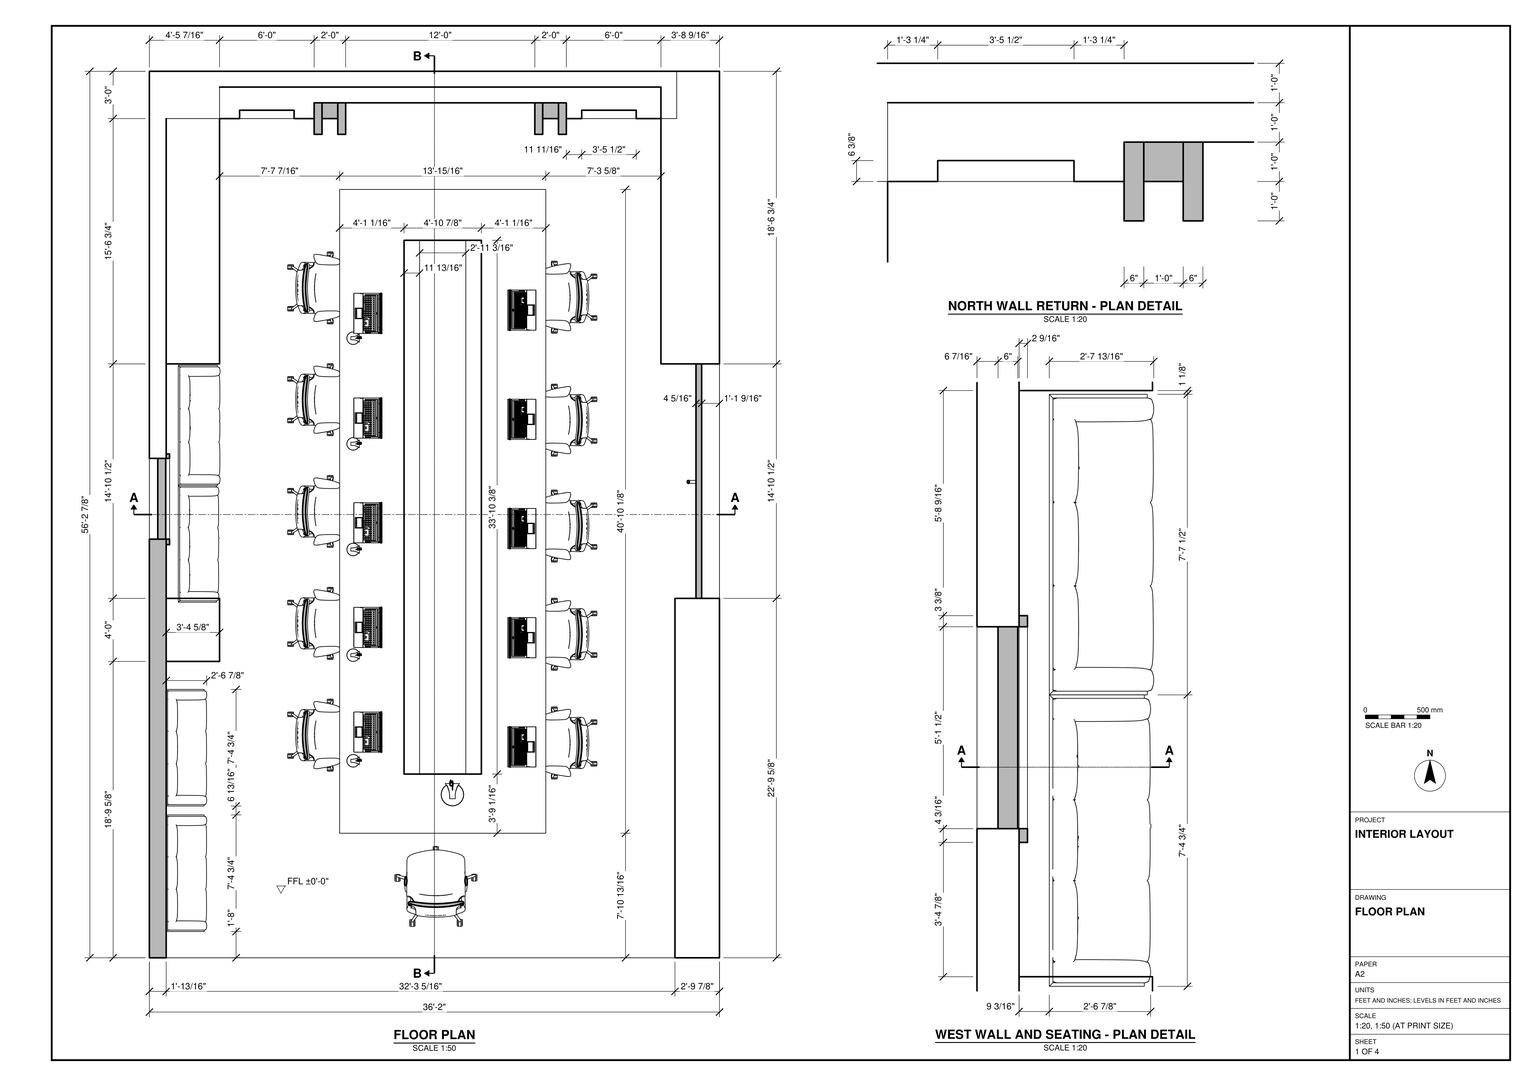
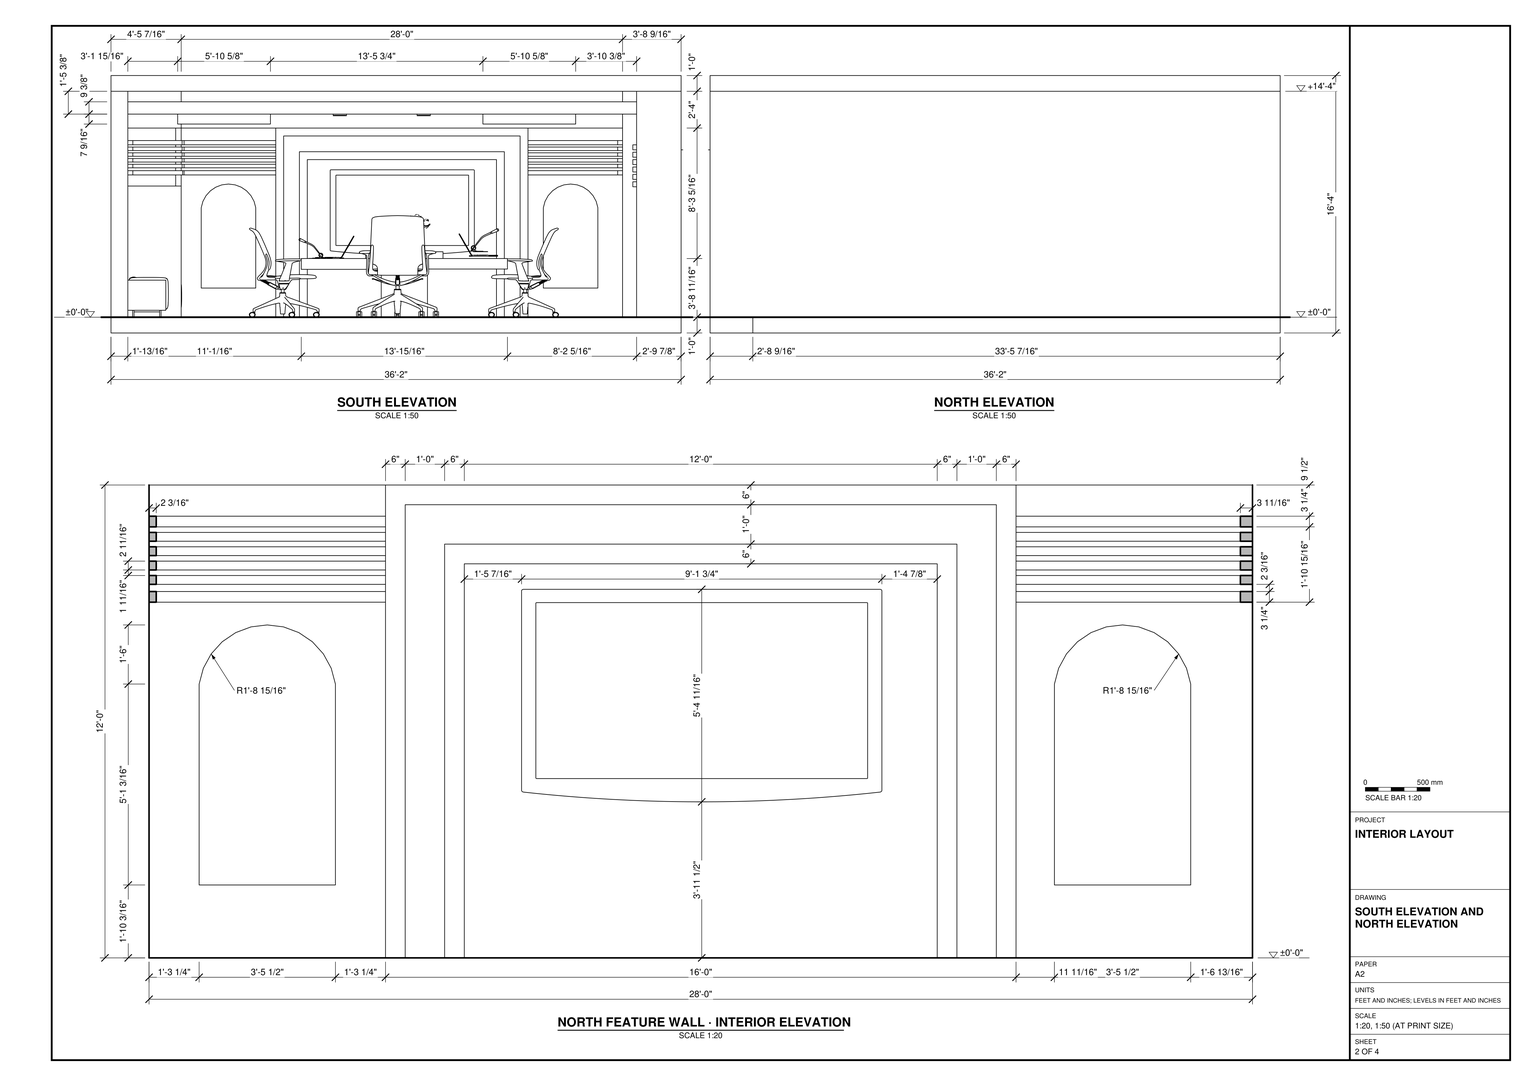
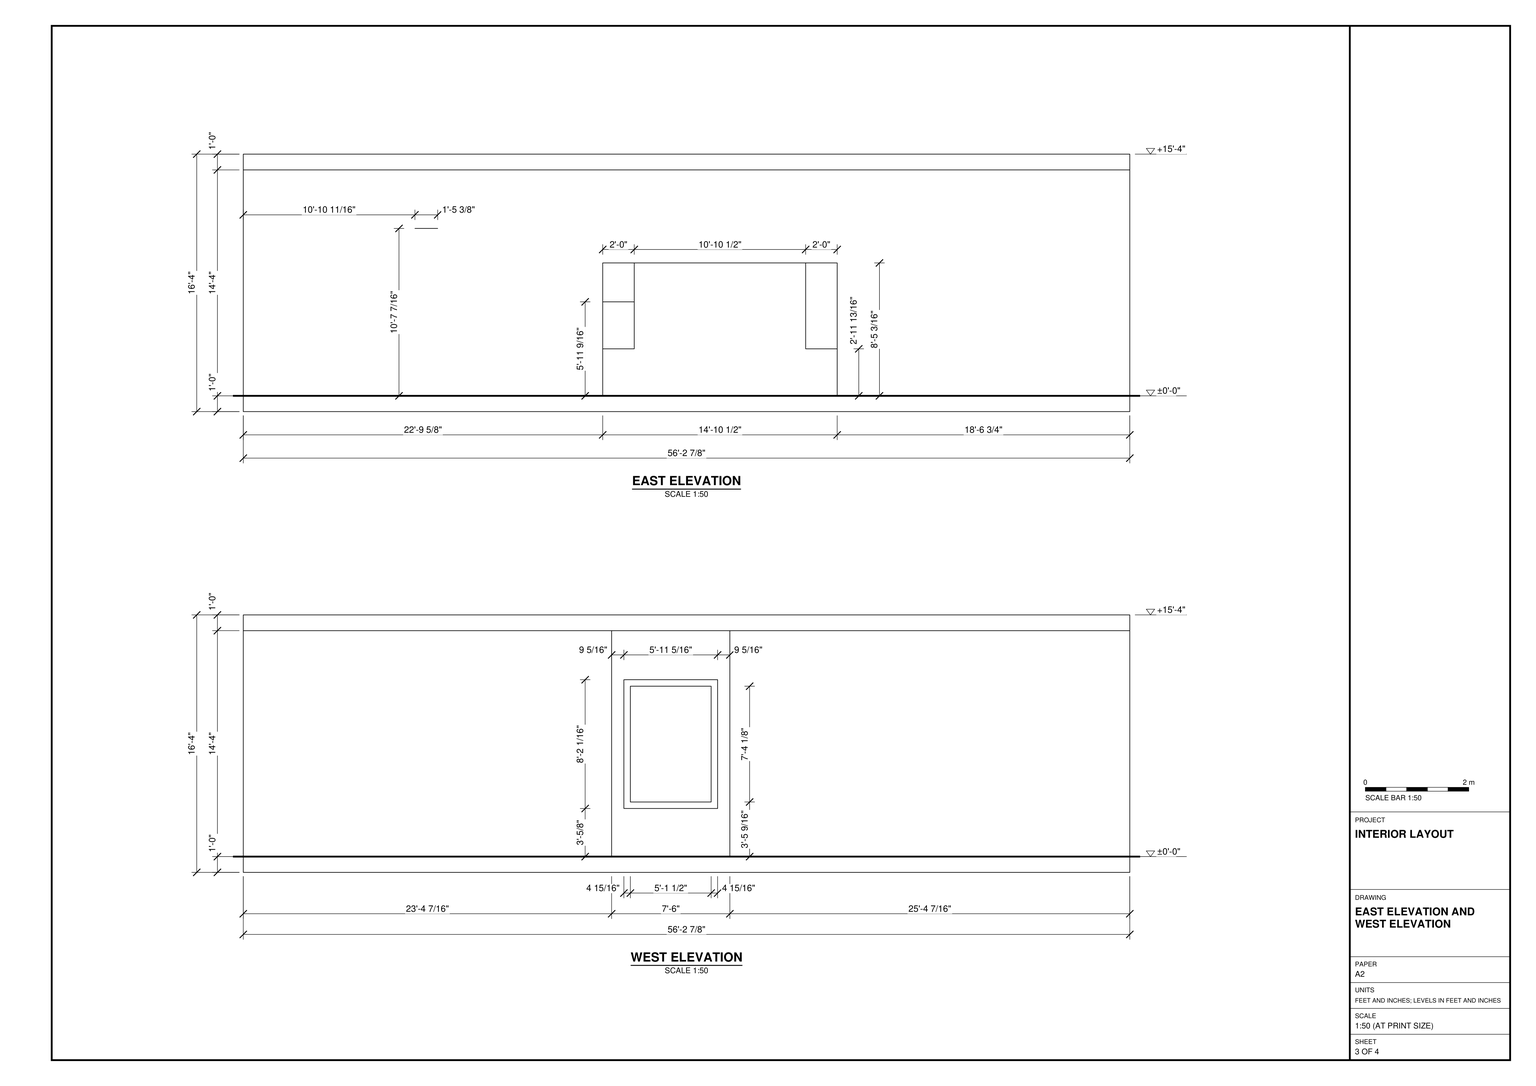
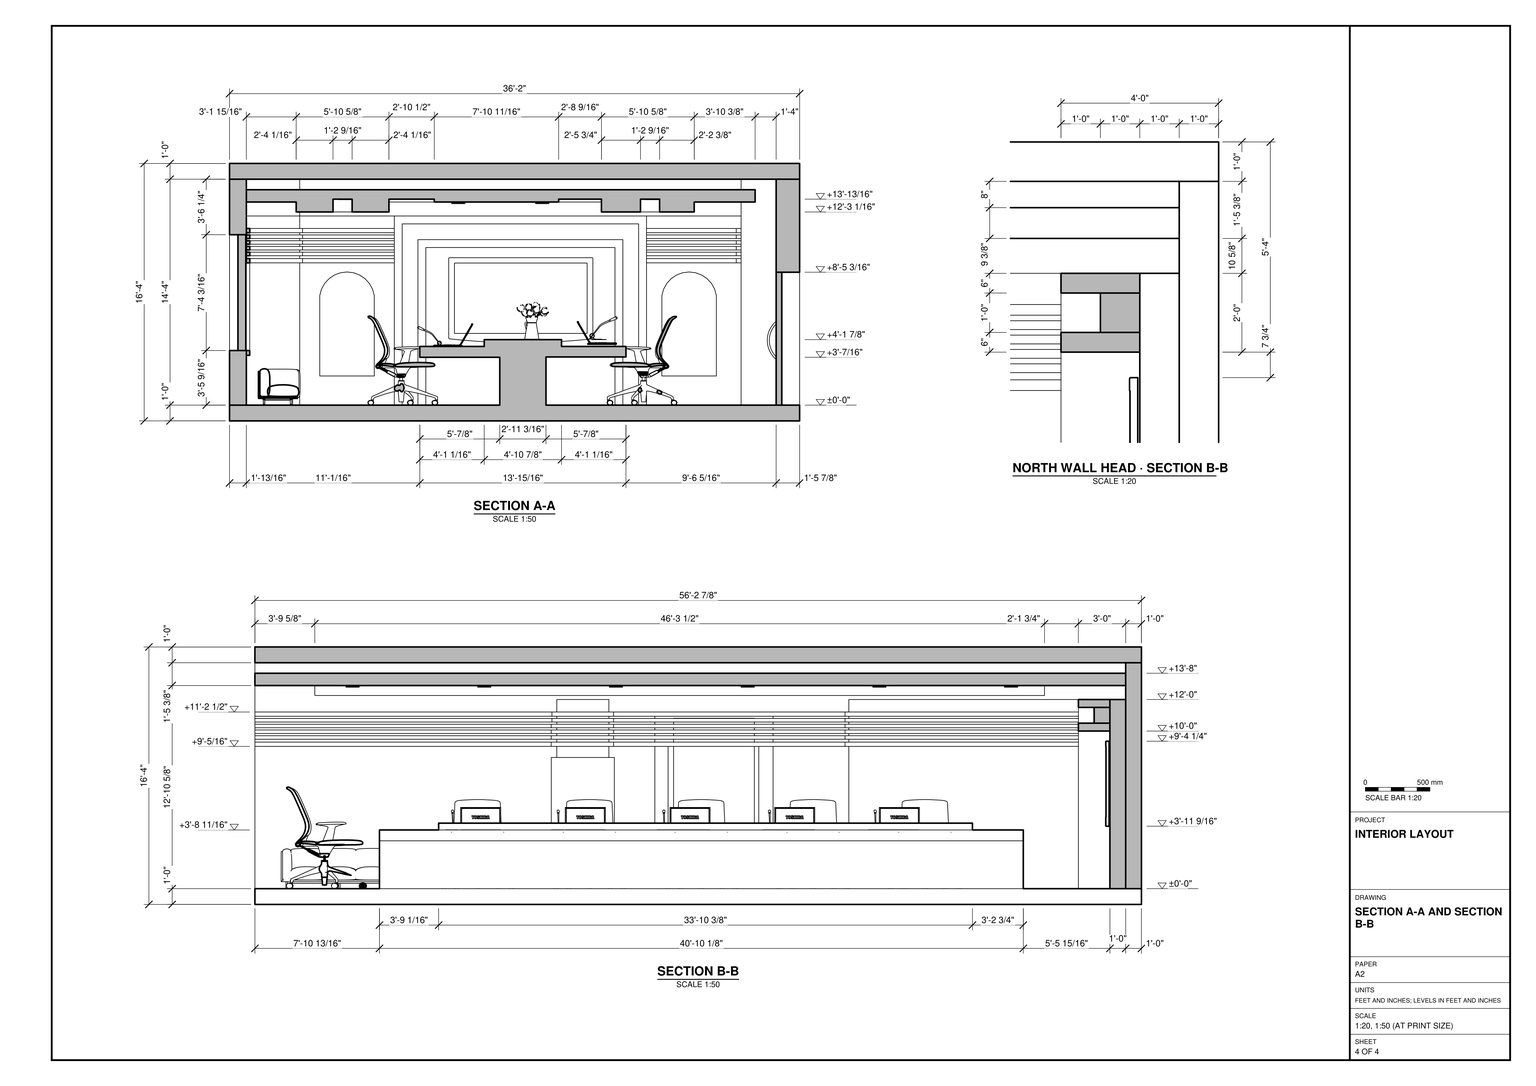
Build the meeting room in SketchUp using task_files/diagram_01.pdf. Work in feet and inches. Set the finished floor at ±0'-0" and make the overall model 36'-2" east to west, 56'-2 7/8" north to south and 16'-4" high, including the floor and overhead slabs.

Use the plan to set out the wall thicknesses and returns. Match the wide east wall opening and the raised, framed opening in the west wall to their respective elevations. On the inside of the north wall, build the stepped rectangular surround for the display. Include the arch-headed panels to either side and the horizontal slats above them.

Place the long meeting table on the north–south axis with its narrower central strip set back from both ends. Arrange five chairs along each long side facing the workstations, with a further chair at the south end facing the display. Fit the sofas along the west wall, preserving the break between the two seating runs shown in plan. Decor and loose items, including computer equipment, may be any suitable library components, for example from 3D Warehouse.

Keep the walls, slabs and each furniture or joinery piece in separate groups or components, and use components for repeated parts. Save one SketchUp model as output_files/meeting_room_with_a_north_display_wall.skp.

# SketchUp Ruby script. Lengths in inches.
U = 1.inch
M = Sketchup.active_model
def pt(a) = Geom::Point3d.new(a.map { |v| v * U })
def face(e, loops, mat)
  f = e.add_face(loops[0].map { |a| pt(a) })
  loops[1..].each { |l| e.add_face(l.map { |a| pt(a) }).erase! }
  f.material = f.back_material = mat if mat
  f
end
# faces: each face lists its corners as indices into pts; further lists are holes
def faces(e, pts, list, mat = nil) = list.each { |f| face(e, (f[0].is_a?(Array) ? f : [f]).map { |l| l.map { |i| pts[i] } }, mat) }
# xy, xz, yz: faces in a plane at the given z, y or x. An outline is a flat list of corners, or four numbers for a rectangle; further outlines are holes
def ring(l) = l.size == 4 ? [[l[0], l[1]], [l[2], l[1]], [l[2], l[3]], [l[0], l[3]]] : l.each_slice(2).to_a
def flat(e, list, mat, &to3) = list.each { |f| face(e, (f[0].is_a?(Array) ? f : [f]).map { |l| ring(l).map { |u, v| to3.(u, v) } }, mat) }
def xy(e, z, list, mat = nil) = flat(e, list, mat) { |x, y| [x, y, z] }
def xz(e, y, list, mat = nil) = flat(e, list, mat) { |x, z| [x, y, z] }
def yz(e, x, list, mat = nil) = flat(e, list, mat) { |y, z| [x, y, z] }
def lines(e, pts, list) = list.each { |a, b| e.add_line(pt(pts[a]), pt(pts[b])) }
# prism: a flat outline (further loops are holes) pulled along v
def prism(e, loops, v, mat = nil)
  f = face(e, loops, mat); d = Geom::Vector3d.new(v.map { |x| x * U })
  f.pushpull(f.normal.samedirection?(d) ? d.length : -d.length)
end
def box(e, o, s, mat = nil) = prism(e, [[o, [o[0] + s[0], o[1], o[2]], [o[0] + s[0], o[1] + s[1], o[2]], [o[0], o[1] + s[1], o[2]]]], [0, 0, s[2]], mat)
def at(x, y, z, deg = 0) = Geom::Transformation.translation(pt([x, y, z])) * Geom::Transformation.rotation(ORIGIN, Z_AXIS, deg.degrees)
def axes(o, x, y, z) = Geom::Transformation.new([*x, 0, *y, 0, *z, 0, *pt(o).to_a, 1])
def part(name) = M.definitions.add(name)
# library, detail: a bought-in or finely detailed component or shape, given as its bounding box
def library(name, o, s) = part(name).tap { |d| box(d.entities, o, s) }
def detail(e, o, s) = box(e.add_group.entities, o, s)
def put(e, d, t, mat = nil) = e.add_instance(d, t).tap { |i| i.material = mat if mat }
def group(e, t, mat = nil) = e.add_group.tap { |g| g.transformation = t; g.material = mat if mat }.entities
root = M.entities
M.materials.add("[Roofing Slate Tan]").color = [198, 174, 127]
M.materials.add("[Translucent Glass Safety]").color = [204, 235, 244]
M.materials["[Translucent Glass Safety]"].alpha = 0.5
M.materials.add("[Wood Bamboo]").color = [170, 101, 41]
M.materials.add("[Wood Cherry Original]").color = [152, 86, 42]
M.materials.add("[Wood Floor Parquet]").color = [127, 77, 33]
c1 = library("of3",[-14.23,-14.05,0],[28.46,27.7,42.45])
c2 = library("Laptop ",[0,0,0],[208.6875,200.66,116.73])
c3 = part("Laptop")
put(c3.entities,c2,at(-0.1875,-132.375,0))
c4 = library("microfono+pc",[-14.125,-4.42,-0.59],[17.32,34.67,27.76])
c5 = library("Pitcher with flowers",[-0.57,-0.27,-0.17],[11.49,12.54,12.88])
c6 = library("Untitled",[82.71,28.87,-11.8125],[39.77,1.97,25.2])
c7 = library("Tlon Light 450 Ceiling 152 006",[-8.86,-8.86,-3.78],[17.72,17.72,3.56])
c8 = library("Group\#1",[0,0,0],[11.09,178.5,101.1875])
c9 = library("Group\#31",[0,0,0],[112.99,39.26,34.22])
xy(root,-12,[[0,0,401.4375,674.875],[401.4375,0,434,674.875]])
xy(root,0,[[0,0,12.8125,0,12.8125,638.875,53.4375,638.875,53.4375,662.875,389.4375,662.875,389.4375,638.875,401.4375,638.875,401.4375,674.875,0,674.875],[[12.8125,0,400.125,0,400.125,273.625,434,273.625,434,452.125,389.4375,452.125,389.4375,638.875,317.4375,638.875,317.4375,626.875,311.4375,626.875,311.4375,638.875,299.4375,638.875,299.4375,626.875,293.4375,626.875,293.4375,650.875,149.4375,650.875,149.4375,626.875,143.4375,626.875,143.4375,638.875,131.4375,638.875,131.4375,626.875,125.4375,626.875,125.4375,638.875,53.4375,638.875,53.4375,452.125,12.8125,452.125,12.8125,273.625,53.4375,273.625,53.4375,225.625,12.8125,225.625],[205.72,94.82,240.91,584.94]],[400.125,0,434,273.625],[12.8125,225.625,53.4375,273.625],[12.8125,452.125,53.4375,638.875],
  [389.4375,452.125,434,452.125,434,674.875,401.4375,674.875,401.4375,638.875,389.4375,638.875],[125.4375,626.875,131.4375,650.875],[143.4375,626.875,149.4375,650.875],[293.4375,626.875,299.4375,650.875],[311.4375,626.875,317.4375,650.875],
  [53.4375,638.875,125.4375,638.875,125.4375,650.875,317.4375,650.875,317.4375,638.875,389.4375,638.875,389.4375,662.875,53.4375,662.875],[131.4375,638.875,143.4375,650.875],[299.4375,638.875,311.4375,650.875]])
xy(root,22.2,[[68.6875,638.875,110.1875,645.25],[329.125,638.875,370.625,645.25]])
xy(root,36.4375,[[144.85,94.82,205.72,584.94]])
xy(root,36.6875,[[240.91,94.82,301.78,584.94]])
xy(root,37.95,[[12.8125,314.53,15.375,383.57]])
xy(root,41.57,[[0,318.71,12.8125,380.2],[12.8125,318.71,15.375,380.2]])
xy(root,44.6875,[[[144.85,94.82,301.78,584.94],[193.89,139.86,252.75,546.22]]],"[Wood Floor Parquet]")
xy(root,49.875,[[193.89,139.86,252.75,546.22]])
xy(root,99.3125,[[397.25,0.6875,400.125,273.625]])
xy(root,99.875,[[12.8125,225.625,53.4375,225.625,53.4375,273.625,12.8125,273.625,12.8125,269.4375,49.25,269.4375,49.25,229.8125,12.8125,229.8125]],"[Wood Floor Parquet]")
xy(root,101.1875,[[416.125,273.625,434,452.125]])
xy(root,103.125,[[397.25,0.6875,400.125,273.625]])
xy(root,104.9375,[[397.25,0,400.125,273.625]])
xy(root,108.3125,[[12.8125,0,12.8125,229.8125,49.25,229.8125,49.25,269.4375,12.8125,269.4375,12.8125,314.53,15.375,314.53,15.375,318.71,12.8125,318.71,12.8125,380.2,15.375,380.2,15.375,383.57,12.8125,383.57,12.8125,452.125,53.4375,452.125,53.4375,638.875,55.625,638.875,55.625,449.25,15.4375,449.25,15.4375,273.0625,54.5625,273.0625,54.5625,225.5625,16.64,225.5625,16.64,0],[12.8125,314.53,15.375,318.71],[385.75,452.125,385.75,634.875,317.4375,634.875,317.4375,638.875,389.4375,638.875,389.4375,452.125],[55.625,634.875,125.4375,638.875]])
xy(root,108.75,[[397.25,0,400.125,273.625]])
xy(root,110.5625,[[397.25,0,400.125,273.625]])
xy(root,111.5625,[[12.8125,0,16.64,0,16.64,225.5625,54.5625,225.5625,54.5625,273.0625,15.4375,273.0625,15.4375,449.25,55.625,449.25,55.625,638.875,53.4375,638.875,53.4375,452.125,12.8125,452.125,12.8125,269.4375,49.25,269.4375,49.25,229.8125,12.8125,229.8125],[385.75,452.125,389.4375,452.125,389.4375,638.875,317.4375,638.875,317.4375,634.875,385.75,634.875],[55.625,634.875,125.4375,638.875]])
xy(root,113.75,[[12.8125,0,12.8125,229.8125,49.25,229.8125,49.25,269.4375,12.8125,269.4375,12.8125,452.125,53.4375,452.125,53.4375,638.875,55.625,638.875,55.625,449.25,15.4375,449.25,15.4375,273.0625,54.125,273.0625,54.125,225.5625,16.64,225.5625,16.64,0],[385.75,452.125,385.75,634.875,317.4375,634.875,317.4375,638.875,389.4375,638.875,389.4375,452.125],[55.625,634.875,125.4375,638.875]])
xy(root,114.375,[[397.25,0,400.125,273.625]])
xy(root,116.1875,[[397.25,0,400.125,273.625]])
xy(root,116.4375,[[12.8125,0,16.64,0,16.64,225.5625,54.125,225.5625,54.125,273.0625,15.4375,273.0625,15.4375,449.25,55.625,449.25,55.625,638.875,53.4375,638.875,53.4375,452.125,12.8125,452.125,12.8125,269.4375,49.25,269.4375,49.25,229.8125,12.8125,229.8125],[385.75,452.125,389.4375,452.125,389.4375,638.875,317.4375,638.875,317.4375,634.875,385.75,634.875],[55.625,634.875,125.4375,638.875]])
xy(root,118.125,[[12.8125,0,12.8125,229.8125,49.25,229.8125,49.25,269.4375,12.8125,269.4375,12.8125,452.125,53.4375,452.125,53.4375,638.875,55.625,638.875,55.625,449.25,15.4375,449.25,15.4375,273.0625,54.125,273.0625,54.125,225.5625,16.64,225.5625,16.64,0],[385.75,452.125,385.75,634.875,317.4375,634.875,317.4375,638.875,389.4375,638.875,389.4375,452.125],[55.625,634.875,125.4375,638.875]])
xy(root,120,[[397.25,0,400.125,273.625]])
xy(root,120,[[149.4375,626.875,293.4375,650.875]],"[Wood Floor Parquet]")
xy(root,120.8125,[[12.8125,0,16.64,0,16.64,225.5625,54.125,225.5625,54.125,273.0625,15.4375,273.0625,15.4375,449.25,55.625,449.25,55.625,638.875,53.4375,638.875,53.4375,452.125,12.8125,452.125,12.8125,269.4375,49.25,269.4375,49.25,229.8125,12.8125,229.8125],[385.75,452.125,389.4375,452.125,389.4375,638.875,317.4375,638.875,317.4375,634.875,385.75,634.875],[55.625,634.875,125.4375,638.875]])
xy(root,121.8125,[[397.25,0,400.125,273.625]])
xy(root,122.5,[[12.8125,0,12.8125,229.8125,49.25,229.8125,49.25,269.4375,12.8125,269.4375,12.8125,452.125,53.4375,452.125,53.4375,638.875,55.625,638.875,55.625,449.25,15.4375,449.25,15.4375,273.0625,54.125,273.0625,54.125,225.5625,16.64,225.5625,16.64,0],[385.75,452.125,385.75,634.875,317.4375,634.875,317.4375,638.875,389.4375,638.875,389.4375,452.125],[55.625,634.875,125.4375,638.875]])
xy(root,125.1875,[[12.8125,0,16.64,0,16.64,225.5625,54.125,225.5625,54.125,273.0625,15.4375,273.0625,15.4375,449.25,55.625,449.25,55.625,638.875,53.4375,638.875,53.4375,452.125,12.8125,452.125,12.8125,269.4375,49.25,269.4375,49.25,229.8125,12.8125,229.8125],[385.75,452.125,389.4375,452.125,389.4375,638.875,317.4375,638.875,317.4375,634.875,385.75,634.875],[55.625,634.875,125.4375,638.875]])
xy(root,125.625,[[397.25,0,400.125,273.625]])
xy(root,126,[[143.4375,638.875,299.4375,650.875]])
xy(root,126,[[143.4375,626.875,299.4375,638.875]],"[Wood Floor Parquet]")
xy(root,126.875,[[12.8125,0,12.8125,229.8125,49.25,229.8125,49.25,269.4375,12.8125,269.4375,12.8125,452.125,53.4375,452.125,53.4375,638.875,55.625,638.875,55.625,449.25,15.4375,449.25,15.4375,273.0625,54.125,273.0625,54.125,226.125,16.64,226.125,16.64,0],[385.75,452.125,385.75,634.875,317.4375,634.875,317.4375,638.875,389.4375,638.875,389.4375,452.125],[55.625,634.875,125.4375,638.875]])
xy(root,127.4375,[[397.25,0,400.125,273.625]])
xy(root,129.5625,[[12.8125,0,16.64,0,16.64,226.125,54.125,226.125,54.125,273.0625,15.4375,273.0625,15.4375,449.25,55.625,449.25,55.625,638.875,53.4375,638.875,53.4375,452.125,12.8125,452.125,12.8125,269.4375,49.25,269.4375,49.25,229.8125,12.8125,229.8125],[385.75,452.125,389.4375,452.125,389.4375,638.875,317.4375,638.875,317.4375,634.875,385.75,634.875],[55.625,634.875,125.4375,638.875]])
xy(root,129.74,[[0,318.71,12.8125,380.2]])
xy(root,131.25,[[12.8125,0,12.8125,229.8125,49.25,229.8125,49.25,269.4375,12.8125,269.4375,12.8125,452.125,53.4375,452.125,53.4375,638.875,55.625,638.875,55.625,449.25,15.4375,449.25,15.4375,273.0625,54.125,273.0625,54.125,226.125,16.64,226.125,16.64,0],[397.25,0,400.125,273.625],[385.75,452.125,385.75,634.875,317.4375,634.875,317.4375,638.875,389.4375,638.875,389.4375,452.125],[55.625,634.875,125.4375,638.875]])
xy(root,134.5,[[12.8125,0,16.64,0,16.64,226.125,54.125,226.125,54.125,273.0625,15.4375,273.0625,15.4375,449.25,55.625,449.25,55.625,638.875,53.4375,638.875,53.4375,452.125,12.8125,452.125,12.8125,269.4375,49.25,269.4375,49.25,229.8125,12.8125,229.8125],[385.75,452.125,389.4375,452.125,389.4375,638.875,317.4375,638.875,317.4375,634.875,385.75,634.875],[55.625,634.875,125.4375,638.875]])
xy(root,138,[[131.4375,626.875,311.4375,638.875],[131.4375,638.875,311.4375,650.875]])
xy(root,144,[[125.4375,626.875,317.4375,650.875]])
xy(root,144,[[12.8125,229.8125,49.25,269.4375],[12.8125,452.125,53.4375,452.125,53.4375,638.875,125.4375,638.875,125.4375,650.875,317.4375,650.875,317.4375,638.875,389.4375,638.875,389.4375,662.875,12.8125,662.875]],"[Wood Floor Parquet]")
xy(root,147.0625,[[[50.75,45.59,121.375,601.09],[78.79,73.64,93.33,251.05],[78.79,312.76,93.33,490.18]],[[283.125,45.59,353.75,601.09],[312.86,312.76,327.39,490.18],[312.86,73.64,327.39,251.05]]])
xy(root,154.625,[[[12.8125,0,400.125,662.875],[50.75,45.59,155.875,601.09],[250.5625,45.59,353.75,601.09]]])
xy(root,156.8125,[[121.375,45.59,155.875,601.09],[250.5625,45.59,283.125,601.09],[78.79,73.64,93.33,251.05],[312.86,73.64,327.39,251.05],[78.79,312.76,93.33,490.18],
  [312.86,312.76,327.39,490.18]],"[Wood Floor Parquet]")
xy(root,164,[[12.8125,0,400.125,662.875]])
xy(root,172,[[0,0,0,674.875,434,674.875,434,0,400.125,0,400.125,273.625,416.125,273.625,416.125,452.125,389.4375,452.125,389.4375,662.875,12.8125,662.875,12.8125,0],[12.8125,0,12.8125,662.875,389.4375,662.875,389.4375,452.125,416.125,452.125,416.125,273.625,400.125,273.625,400.125,0]])
xy(root,184,[[0,0,434,674.875]])
xz(root,0,[[0,-12,434,0],[0,0,12.8125,172],[400.125,0,434,172],[397.25,104.9375,400.125,108.75],[12.8125,108.3125,16.64,111.5625],
  [397.25,110.5625,400.125,114.375],[12.8125,113.75,16.64,116.4375],[397.25,116.1875,400.125,120],[12.8125,118.125,16.64,120.8125],[397.25,121.8125,400.125,125.625],
  [12.8125,122.5,16.64,125.1875],[12.8125,126.875,16.64,129.5625],[397.25,127.4375,400.125,131.25],[12.8125,131.25,16.64,134.5],[12.8125,154.625,400.125,164],
  [0,172,434,184]])
xz(root,0.6875,[[397.25,99.3125,400.125,103.125]])
xz(root,45.59,[[50.75,147.0625,121.375,154.625],[283.125,147.0625,353.75,154.625],[121.375,154.625,155.875,156.8125],[250.5625,154.625,283.125,156.8125]])
xz(root,73.64,[[78.79,147.0625,93.33,156.8125],[312.86,147.0625,327.39,156.8125]])
xz(root,94.82,[[205.72,0,240.91,0,240.91,36.6875,301.78,36.6875,301.78,44.6875,144.85,44.6875,144.85,36.4375,205.72,36.4375]],"[Wood Floor Parquet]")
xz(root,139.86,[[193.89,44.6875,252.75,49.875]])
xz(root,225.5625,[[16.64,108.3125,54.5625,111.5625],[16.64,113.75,54.125,116.4375],[16.64,118.125,54.125,120.8125],[16.64,122.5,54.125,125.1875]])
xz(root,225.625,[[12.8125,0,53.4375,99.875]],"[Wood Floor Parquet]")
xz(root,226.125,[[16.64,126.875,54.125,129.5625],[16.64,131.25,54.125,134.5]])
xz(root,229.8125,[[12.8125,111.5625,49.25,113.75],[12.8125,116.4375,49.25,118.125],[12.8125,120.8125,49.25,122.5],[12.8125,125.1875,49.25,126.875],[12.8125,129.5625,49.25,131.25]])
xz(root,229.8125,[[12.8125,99.875,49.25,108.3125],[12.8125,134.5,49.25,144]],"[Wood Floor Parquet]")
xz(root,251.05,[[78.79,147.0625,93.33,156.8125],[312.86,147.0625,327.39,156.8125]],"[Wood Floor Parquet]")
xz(root,269.4375,[[12.8125,99.875,49.25,108.3125],[12.8125,111.5625,49.25,113.75],[12.8125,116.4375,49.25,118.125],[12.8125,120.8125,49.25,122.5],[12.8125,125.1875,49.25,126.875],
  [12.8125,129.5625,49.25,131.25],[12.8125,134.5,49.25,144]])
xz(root,273.0625,[[15.4375,108.3125,54.5625,111.5625],[15.4375,113.75,54.125,116.4375],[15.4375,118.125,54.125,120.8125],[15.4375,122.5,54.125,125.1875],[15.4375,126.875,54.125,129.5625],
  [15.4375,131.25,54.125,134.5]])
xz(root,273.625,[[12.8125,0,53.4375,99.875],[400.125,0,400.125,172,416.125,172,416.125,101.1875,434,101.1875,434,0],[397.25,99.3125,400.125,103.125],[397.25,104.9375,400.125,108.75],[397.25,110.5625,400.125,114.375],
  [397.25,116.1875,400.125,120],[397.25,121.8125,400.125,125.625],[397.25,127.4375,400.125,131.25]])
xz(root,312.76,[[78.79,147.0625,93.33,156.8125],[312.86,147.0625,327.39,156.8125]])
xz(root,314.53,[[12.8125,37.95,15.375,108.3125]])
xz(root,318.71,[[0,41.57,12.8125,129.74],[12.8125,41.57,15.375,108.3125]])
xz(root,380.2,[[0,41.57,12.8125,129.74],[12.8125,41.57,15.375,108.3125]])
xz(root,383.57,[[12.8125,37.95,15.375,108.3125]])
xz(root,449.25,[[15.4375,108.3125,55.625,111.5625],[15.4375,113.75,55.625,116.4375],[15.4375,118.125,55.625,120.8125],[15.4375,122.5,55.625,125.1875],[15.4375,126.875,55.625,129.5625],
  [15.4375,131.25,55.625,134.5]])
xz(root,452.125,[[12.8125,108.3125,53.4375,111.5625],[385.75,108.3125,389.4375,111.5625],[12.8125,111.5625,53.4375,113.75],[12.8125,113.75,53.4375,116.4375],[385.75,113.75,389.4375,116.4375],
  [12.8125,116.4375,53.4375,118.125],[12.8125,118.125,53.4375,120.8125],[385.75,118.125,389.4375,120.8125],[12.8125,120.8125,53.4375,122.5],[12.8125,122.5,53.4375,125.1875],
  [385.75,122.5,389.4375,125.1875],[12.8125,125.1875,53.4375,126.875],[12.8125,126.875,53.4375,129.5625],[385.75,126.875,389.4375,129.5625],[12.8125,129.5625,53.4375,131.25],
  [12.8125,131.25,53.4375,134.5],[385.75,131.25,389.4375,134.5]])
xz(root,452.125,[[12.8125,0,53.4375,108.3125],[389.4375,0,434,0,434,101.1875,416.125,101.1875,416.125,172,389.4375,172],[12.8125,134.5,53.4375,144]],"[Wood Floor Parquet]")
xz(root,490.18,[[78.79,147.0625,93.33,156.8125],[312.86,147.0625,327.39,156.8125]],"[Wood Floor Parquet]")
xz(root,546.22,[[193.89,44.6875,252.75,49.875]])
xz(root,584.94,[[205.72,0,205.72,36.4375,144.85,36.4375,144.85,44.6875,301.78,44.6875,301.78,36.6875,240.91,36.6875,240.91,0]])
xz(root,601.09,[[50.75,147.0625,121.375,154.625],[283.125,147.0625,353.75,154.625]])
xz(root,601.09,[[121.375,154.625,155.875,156.8125],[250.5625,154.625,283.125,156.8125]],"[Wood Floor Parquet]")
xz(root,626.875,[[125.4375,0,131.4375,0,131.4375,138,311.4375,138,311.4375,0,317.4375,0,317.4375,144,125.4375,144]])
xz(root,626.875,[[143.4375,0,149.4375,0,149.4375,120,293.4375,120,293.4375,0,299.4375,0,299.4375,126,143.4375,126]],"[Wood Floor Parquet]")
xz(root,634.875,[[55.625,108.3125,125.4375,111.5625],[317.4375,108.3125,385.75,111.5625],[55.625,113.75,125.4375,116.4375],[317.4375,113.75,385.75,116.4375],[55.625,118.125,125.4375,120.8125],
  [317.4375,118.125,385.75,120.8125],[55.625,122.5,125.4375,125.1875],[317.4375,122.5,385.75,125.1875],[55.625,126.875,125.4375,129.5625],[317.4375,126.875,385.75,129.5625],
  [55.625,131.25,125.4375,134.5],[317.4375,131.25,385.75,134.5]])
xz(root,638.875,[[53.4375,108.3125,55.625,111.5625],[53.4375,111.5625,125.4375,113.75],[317.4375,111.5625,389.4375,113.75],[53.4375,113.75,55.625,116.4375],[53.4375,116.4375,125.4375,118.125],
  [317.4375,116.4375,389.4375,118.125],[53.4375,118.125,55.625,120.8125],[53.4375,120.8125,125.4375,122.5],[317.4375,120.8125,389.4375,120.8125,389.4375,122.5,317.125,122.5,317.125,125.1875,389.4375,125.1875,389.4375,126.875,317.4375,126.875],[53.4375,122.5,55.625,125.1875],
  [317.125,122.5,317.4375,125.1875],[53.4375,125.1875,125.4375,126.875],[53.4375,126.875,55.625,129.5625],[53.4375,129.5625,125.4375,131.25],[317.4375,129.5625,389.4375,131.25],
  [53.4375,131.25,55.625,134.5]])
xz(root,638.875,[[131.4375,0,143.4375,0,143.4375,126,299.4375,126,299.4375,0,311.4375,0,311.4375,138,131.4375,138]],"[Roofing Slate Tan]")
xz(root,638.875,[[[53.4375,0,125.4375,108.3125],[68.6875,22.2,68.6875,83.39,69.97,88.2,72.35,92.57,75.7,96.26,79.82,99.06,84.49,100.8,89.4375,101.39,94.38,100.8,99.05,99.06,103.17,96.26,106.52,92.57,108.9,88.2,110.1875,83.39,110.1875,22.2]],[[317.4375,0,389.4375,108.3125],[329.125,22.2,329.125,83.39,330.41,88.2,332.79,92.57,336.14,96.26,340.26,99.06,344.93,100.8,349.875,101.39,354.82,100.8,359.49,99.06,363.61,96.26,366.96,92.57,369.34,88.2,370.625,83.39,370.625,22.2]],[53.4375,134.5,125.4375,144],[317.4375,134.5,389.4375,144]],"[Wood Floor Parquet]")
xz(root,645.25,[[68.6875,22.2,110.1875,22.2,110.1875,83.39,108.9,88.2,106.52,92.57,103.17,96.26,99.05,99.06,94.38,100.8,89.4375,101.39,84.49,100.8,79.82,99.06,75.7,96.26,72.35,92.57,69.97,88.2,68.6875,83.39],[329.125,22.2,370.625,22.2,370.625,83.39,369.34,88.2,366.96,92.57,363.61,96.26,359.49,99.06,354.82,100.8,349.875,101.39,344.93,100.8,340.26,99.06,336.14,96.26,332.79,92.57,330.41,88.2,329.125,83.39]])
xz(root,650.875,[[125.4375,0,125.4375,144,317.4375,144,317.4375,0,311.4375,0,311.4375,138,131.4375,138,131.4375,0],[131.4375,0,131.4375,138,311.4375,138,311.4375,0,299.4375,0,299.4375,126,143.4375,126,143.4375,0],[143.4375,0,143.4375,126,299.4375,126,299.4375,0,293.4375,0,293.4375,120,149.4375,120,149.4375,0]])
xz(root,650.875,[[149.4375,0,293.4375,120]],"[Wood Cherry Original]")
xz(root,662.875,[[53.4375,0,389.4375,144],[12.8125,144,53.4375,154.625],[12.8125,154.625,53.4375,164],[389.4375,154.625,400.125,164],[12.8125,164,53.4375,172]])
xz(root,662.875,[[53.4375,144,389.4375,154.625],[53.4375,154.625,389.4375,164],[53.4375,164,389.4375,172]],"[Wood Floor Parquet]")
xz(root,674.875,[[0,-12,401.4375,0],[401.4375,-12,434,0],[0,0,434,172],[0,172,434,184]])
yz(root,0,[[0,-12,674.875,0],[0,0,304.46,172],[[304.46,0,394.46,172],[313.78,36.63,385.13,134.68]],[394.46,0,674.875,172],[[313.78,36.63,385.13,134.68],[318.71,41.57,380.2,129.74]],
  [0,172,674.875,184]])
yz(root,12.8125,[[225.625,0,225.625,99.875,229.8125,99.875,229.8125,144,269.4375,144,269.4375,134.5,273.625,134.5,273.625,131.25,269.4375,131.25,269.4375,129.5625,273.625,129.5625,273.625,126.875,269.4375,126.875,269.4375,125.1875,273.625,125.1875,273.625,122.5,269.4375,122.5,269.4375,120.8125,273.625,120.8125,273.625,118.125,269.4375,118.125,269.4375,116.4375,273.625,116.4375,273.625,113.75,269.4375,113.75,269.4375,111.5625,273.625,111.5625,273.625,108.3125,269.4375,108.3125,269.4375,99.875,273.625,99.875,273.625,0],[273.625,0,304.46,0,304.46,111.5625,273.625,111.5625,273.625,108.3125,304.46,108.3125,269.4375,108.3125,269.4375,99.875,273.625,99.875],[304.46,0,394.46,0,394.46,108.3125,383.57,108.3125,383.57,37.95,314.53,37.95,314.53,108.3125,304.46,108.3125],[452.125,0,638.875,144],[314.53,37.95,314.53,108.3125,318.71,108.3125,318.71,41.57,380.2,41.57,380.2,108.3125,383.57,108.3125,383.57,37.95],
  [304.46,108.3125,318.71,111.5625],[318.71,108.3125,380.2,111.5625],[380.2,108.3125,394.46,111.5625],[0,111.5625,229.8125,113.75],[269.4375,111.5625,304.46,113.75],
  [304.46,111.5625,318.71,113.75],[318.71,111.5625,380.2,113.75],[380.2,111.5625,394.46,113.75],[394.46,111.5625,452.125,113.75],[273.625,113.75,304.46,116.4375],
  [[273.625,113.75,452.125,113.75,452.125,116.4375,394.46,116.4375,394.46,118.125,452.125,118.125,452.125,120.8125,394.46,120.8125,394.46,122.5,452.125,122.5,452.125,125.1875,394.46,125.1875,394.46,126.875,452.125,126.875,452.125,129.5625,394.46,129.5625,394.46,131.25,304.46,131.25,304.46,129.5625,273.625,129.5625,273.625,126.875,304.46,126.875,304.46,125.1875,273.625,125.1875,273.625,122.5,304.46,122.5,304.46,120.8125,273.625,120.8125,273.625,118.125,304.46,118.125,304.46,116.4375,273.625,116.4375],[318.71,126.875,394.46,129.5625],[304.46,122.5,380.2,125.1875],[318.71,118.125,394.46,120.8125]],[304.46,113.75,318.71,116.4375],[318.71,113.75,380.2,116.4375],[380.2,113.75,394.46,116.4375],[394.46,113.75,452.125,116.4375],
  [0,116.4375,229.8125,118.125],[269.4375,116.4375,304.46,118.125],[304.46,116.4375,318.71,118.125],[318.71,116.4375,380.2,118.125],[380.2,116.4375,394.46,118.125],
  [394.46,116.4375,452.125,118.125],[273.625,118.125,304.46,120.8125],[304.46,118.125,318.71,120.8125],[318.71,118.125,380.2,120.8125],[318.71,118.125,380.2,122.5],
  [380.2,118.125,394.46,120.8125],[394.46,118.125,452.125,120.8125],[0,120.8125,229.8125,122.5],[269.4375,120.8125,304.46,122.5],[304.46,120.8125,318.71,122.5],
  [318.71,120.8125,380.2,122.5],[380.2,120.8125,394.46,122.5],[394.46,120.8125,452.125,122.5],[273.625,122.5,304.46,125.1875],[304.46,122.5,318.71,125.1875],
  [318.71,122.5,380.2,125.1875],[380.2,122.5,394.46,125.1875],[394.46,122.5,452.125,125.1875],[0,125.1875,229.8125,126.875],[269.4375,125.1875,304.46,126.875],
  [304.46,125.1875,318.71,126.875],[318.71,125.1875,380.2,126.875],[380.2,125.1875,394.46,126.875],[394.46,125.1875,452.125,126.875],[273.625,126.875,304.46,129.5625],
  [304.46,126.875,318.71,129.5625],[318.71,126.875,380.2,129.5625],[380.2,126.875,394.46,129.5625],[394.46,126.875,452.125,129.5625],[0,129.5625,229.8125,131.25],
  [269.4375,129.5625,304.46,131.25],[304.46,129.5625,318.71,129.5625,318.71,129.74,380.2,129.74,380.2,129.5625,394.46,129.5625,394.46,131.25,304.46,131.25],[318.71,129.5625,380.2,129.74],[394.46,129.5625,452.125,131.25],[273.625,131.25,304.46,134.5],
  [304.46,131.25,394.46,134.5],[394.46,131.25,452.125,134.5],[0,154.625,662.875,164]])
yz(root,12.8125,[[0,0,225.625,0,225.625,99.875,229.8125,99.875,229.8125,108.3125,0,108.3125],[394.46,0,452.125,0,452.125,108.3125,394.46,108.3125,452.125,108.3125,452.125,111.5625,394.46,111.5625],[0,134.5,229.8125,134.5,229.8125,144,269.4375,144,269.4375,134.5,452.125,134.5,452.125,144,662.875,144,662.875,154.625,0,154.625],[0,164,662.875,172]],"[Wood Floor Parquet]")
yz(root,15.375,[[314.53,37.95,383.57,37.95,383.57,108.3125,380.2,108.3125,380.2,41.57,318.71,41.57,318.71,108.3125,314.53,108.3125]])
yz(root,15.4375,[[273.0625,108.3125,449.25,111.5625],[273.0625,113.75,449.25,116.4375],[273.0625,118.125,449.25,120.8125],[273.0625,122.5,449.25,125.1875],[273.0625,126.875,449.25,129.5625],
  [273.0625,131.25,449.25,134.5]])
yz(root,16.64,[[0,108.3125,225.5625,111.5625],[0,113.75,225.5625,116.4375],[0,118.125,225.5625,120.8125],[0,122.5,225.5625,125.1875],[0,126.875,226.125,129.5625],
  [0,131.25,226.125,134.5]])
yz(root,49.25,[[229.8125,111.5625,269.4375,113.75],[229.8125,116.4375,269.4375,118.125],[229.8125,120.8125,269.4375,122.5],[229.8125,125.1875,269.4375,126.875],[229.8125,129.5625,269.4375,131.25]])
yz(root,49.25,[[229.8125,99.875,269.4375,108.3125],[229.8125,134.5,269.4375,144]],"[Wood Floor Parquet]")
yz(root,50.75,[[45.59,147.0625,601.09,154.625]])
yz(root,53.4375,[[452.125,108.3125,638.875,111.5625],[452.125,111.5625,638.875,113.75],[452.125,113.75,638.875,116.4375],[452.125,116.4375,638.875,118.125],[452.125,118.125,638.875,120.8125],
  [452.125,120.8125,638.875,122.5],[452.125,122.5,638.875,125.1875],[452.125,125.1875,638.875,126.875],[452.125,126.875,638.875,129.5625],[452.125,129.5625,638.875,131.25],
  [452.125,131.25,638.875,134.5]])
yz(root,53.4375,[[225.625,0,273.625,99.875],[452.125,0,638.875,108.3125],[452.125,134.5,638.875,144]],"[Wood Floor Parquet]")
yz(root,54.125,[[225.5625,113.75,273.0625,116.4375],[225.5625,118.125,273.0625,120.8125],[225.5625,122.5,273.0625,125.1875],[226.125,126.875,273.0625,129.5625],[226.125,131.25,273.0625,134.5]])
yz(root,54.5625,[[225.5625,108.3125,273.0625,111.5625]])
yz(root,55.625,[[449.25,108.3125,634.875,111.5625],[634.875,108.3125,638.875,111.5625],[449.25,113.75,634.875,116.4375],[634.875,113.75,638.875,116.4375],[449.25,118.125,634.875,120.8125],
  [634.875,118.125,638.875,120.8125],[449.25,122.5,634.875,125.1875],[634.875,122.5,638.875,125.1875],[449.25,126.875,634.875,129.5625],[634.875,126.875,638.875,129.5625],
  [449.25,131.25,634.875,134.5],[634.875,131.25,638.875,134.5]])
yz(root,68.6875,[[638.875,22.2,645.25,83.39]])
yz(root,78.79,[[73.64,147.0625,251.05,156.8125],[312.76,147.0625,490.18,156.8125]],"[Wood Floor Parquet]")
yz(root,93.33,[[73.64,147.0625,251.05,156.8125],[312.76,147.0625,490.18,156.8125]],"[Wood Floor Parquet]")
yz(root,110.1875,[[638.875,22.2,645.25,83.39]])
yz(root,121.375,[[45.59,147.0625,601.09,156.8125]])
yz(root,125.4375,[[626.875,0,626.875,144,638.875,144,638.875,134.5,634.875,134.5,634.875,131.25,638.875,131.25,638.875,129.5625,634.875,129.5625,634.875,126.875,638.875,126.875,638.875,125.1875,634.875,125.1875,634.875,122.5,638.875,122.5,638.875,120.8125,634.875,120.8125,634.875,118.125,638.875,118.125,638.875,116.4375,634.875,116.4375,634.875,113.75,638.875,113.75,638.875,111.5625,634.875,111.5625,634.875,108.3125,638.875,108.3125,638.875,0],[638.875,0,638.875,108.3125,634.875,108.3125,634.875,111.5625,638.875,111.5625,638.875,113.75,634.875,113.75,634.875,116.4375,638.875,116.4375,638.875,118.125,634.875,118.125,634.875,120.8125,638.875,120.8125,638.875,122.5,634.875,122.5,634.875,125.1875,638.875,125.1875,638.875,126.875,634.875,126.875,634.875,129.5625,638.875,129.5625,638.875,131.25,634.875,131.25,634.875,134.5,638.875,134.5,638.875,144,650.875,144,650.875,0]])
yz(root,131.4375,[[626.875,0,638.875,138],[638.875,0,650.875,138]])
yz(root,143.4375,[[638.875,0,650.875,126]])
yz(root,143.4375,[[626.875,0,638.875,126]],"[Wood Floor Parquet]")
yz(root,144.85,[[94.82,36.4375,584.94,44.6875]],"[Wood Floor Parquet]")
yz(root,149.4375,[[626.875,0,650.875,120]],"[Wood Floor Parquet]")
yz(root,155.875,[[45.59,154.625,601.09,156.8125]],"[Wood Floor Parquet]")
yz(root,193.89,[[139.86,44.6875,546.22,49.875]])
yz(root,205.72,[[94.82,0,584.94,36.4375]],"[Wood Floor Parquet]")
yz(root,240.91,[[94.82,0,584.94,36.6875]],"[Wood Floor Parquet]")
yz(root,250.5625,[[45.59,154.625,601.09,156.8125]],"[Wood Floor Parquet]")
yz(root,252.75,[[139.86,44.6875,546.22,49.875]])
yz(root,283.125,[[45.59,147.0625,601.09,156.8125]])
yz(root,293.4375,[[626.875,0,650.875,120]],"[Wood Floor Parquet]")
yz(root,299.4375,[[638.875,0,650.875,126]])
yz(root,299.4375,[[626.875,0,638.875,126]],"[Wood Floor Parquet]")
yz(root,301.78,[[94.82,36.6875,584.94,44.6875]],"[Wood Floor Parquet]")
yz(root,311.4375,[[626.875,0,638.875,138],[638.875,0,650.875,138]])
yz(root,312.86,[[73.64,147.0625,251.05,156.8125],[312.76,147.0625,490.18,156.8125]],"[Wood Floor Parquet]")
yz(root,317.4375,[[626.875,0,638.875,0,638.875,108.3125,634.875,108.3125,634.875,111.5625,638.875,111.5625,638.875,113.75,634.875,113.75,634.875,116.4375,638.875,116.4375,638.875,118.125,634.875,118.125,634.875,120.8125,638.875,120.8125,638.875,122.5,634.875,122.5,634.875,125.1875,638.875,125.1875,638.875,126.875,634.875,126.875,634.875,129.5625,638.875,129.5625,638.875,131.25,634.875,131.25,634.875,134.5,638.875,134.5,638.875,144,626.875,144],[638.875,0,650.875,0,650.875,144,638.875,144,638.875,134.5,634.875,134.5,634.875,131.25,638.875,131.25,638.875,129.5625,634.875,129.5625,634.875,126.875,638.875,126.875,638.875,120.8125,634.875,120.8125,634.875,118.125,638.875,118.125,638.875,116.4375,634.875,116.4375,634.875,113.75,638.875,113.75,638.875,111.5625,634.875,111.5625,634.875,108.3125,638.875,108.3125],[634.875,122.5,638.875,125.1875]])
yz(root,327.39,[[73.64,147.0625,251.05,156.8125],[312.76,147.0625,490.18,156.8125]],"[Wood Floor Parquet]")
yz(root,329.125,[[638.875,22.2,645.25,83.39]])
yz(root,353.75,[[45.59,147.0625,601.09,154.625]])
yz(root,370.625,[[638.875,22.2,645.25,83.39]])
yz(root,385.75,[[452.125,108.3125,634.875,111.5625],[452.125,113.75,634.875,116.4375],[452.125,118.125,634.875,120.8125],[452.125,122.5,634.875,125.1875],[452.125,126.875,634.875,129.5625],
  [452.125,131.25,634.875,134.5]])
yz(root,389.4375,[[638.875,0,638.875,108.3125,452.125,108.3125,452.125,111.5625,638.875,111.5625,638.875,113.75,452.125,113.75,452.125,116.4375,638.875,116.4375,638.875,118.125,452.125,118.125,452.125,120.8125,638.875,120.8125,638.875,122.5,452.125,122.5,452.125,125.1875,638.875,125.1875,638.875,126.875,452.125,126.875,452.125,129.5625,638.875,129.5625,638.875,131.25,452.125,131.25,452.125,134.5,638.875,134.5,638.875,144,662.875,144,662.875,0],[452.125,111.5625,638.875,113.75],[452.125,116.4375,638.875,118.125],[452.125,120.8125,638.875,122.5],[452.125,125.1875,638.875,126.875],
  [452.125,129.5625,638.875,131.25]])
yz(root,389.4375,[[452.125,0,638.875,108.3125],[452.125,134.5,452.125,172,662.875,172,662.875,144,638.875,144,638.875,134.5]],"[Wood Floor Parquet]")
yz(root,397.25,[[0.6875,99.3125,273.625,103.125],[0,104.9375,273.625,108.75],[0,110.5625,273.625,114.375],[0,116.1875,273.625,120],[0,121.8125,273.625,125.625],
  [0,127.4375,273.625,131.25]])
yz(root,400.125,[[0,99.3125,0.6875,103.125],[0.6875,99.3125,273.625,103.125],[0,103.125,273.625,104.9375],[0,104.9375,273.625,108.75],[0,108.75,273.625,110.5625],
  [0,110.5625,273.625,114.375],[0,114.375,273.625,116.1875],[0,116.1875,273.625,120],[0,120,273.625,121.8125],[0,121.8125,273.625,125.625],
  [0,125.625,273.625,127.4375],[0,127.4375,273.625,131.25],[0,154.625,273.625,164],[273.625,154.625,452.125,164],[452.125,154.625,662.875,164]])
yz(root,400.125,[[0,0,273.625,99.3125],[0,131.25,273.625,154.625],[0,164,273.625,172]],"[Wood Floor Parquet]")
yz(root,416.125,[[273.625,101.1875,452.125,172]],"[Wood Bamboo]")
yz(root,434,[[0,-12,674.875,0],[0,0,273.625,0,273.625,101.1875,452.125,101.1875,452.125,0,674.875,0,674.875,172,0,172],[0,172,674.875,184]])
p = [[69.97,638.875,88.2],[68.6875,638.875,83.39],[68.6875,645.25,83.39],[69.97,645.25,88.2],[110.1875,638.875,83.39],[108.9,638.875,88.2],
  [108.9,645.25,88.2],[110.1875,645.25,83.39],[330.41,638.875,88.2],[329.125,638.875,83.39],[329.125,645.25,83.39],[330.41,645.25,88.2],
  [370.625,638.875,83.39],[369.34,638.875,88.2],[369.34,645.25,88.2],[370.625,645.25,83.39],[72.35,638.875,92.57],[72.35,645.25,92.57],
  [106.52,638.875,92.57],[106.52,645.25,92.57],[332.79,638.875,92.57],[332.79,645.25,92.57],[366.96,638.875,92.57],[366.96,645.25,92.57],
  [75.7,638.875,96.26],[75.7,645.25,96.26],[103.17,638.875,96.26],[103.17,645.25,96.26],[336.14,638.875,96.26],[336.14,645.25,96.26],
  [363.61,638.875,96.26],[363.61,645.25,96.26],[79.82,638.875,99.06],[79.82,645.25,99.06],[99.05,638.875,99.06],[99.05,645.25,99.06],
  [340.26,638.875,99.06],[340.26,645.25,99.06],[359.49,638.875,99.06],[359.49,645.25,99.06],[84.49,638.875,100.8],[84.49,645.25,100.8],
  [94.38,638.875,100.8],[94.38,645.25,100.8],[344.93,638.875,100.8],[344.93,645.25,100.8],[354.82,638.875,100.8],[354.82,645.25,100.8],
  [89.4375,638.875,101.39],[89.4375,645.25,101.39],[349.875,638.875,101.39],[349.875,645.25,101.39],[416.23,130.68,127.4375],[416.23,148.05,127.4375],
  [400.83,148.05,127.4375],[400.83,130.68,127.4375],[435.33,130.66,127.4375],[435.33,148.02,127.4375],[419.93,148.02,127.4375],[419.93,130.66,127.4375]]
faces(root,p,[[0,1,2,3],[4,5,6,7],[8,9,10,11],[12,13,14,15],[16,0,3,17],[5,18,19,6],[20,8,11,21],[13,22,23,14],
  [24,16,17,25],[18,26,27,19],[28,20,21,29],[22,30,31,23],[32,24,25,33],[26,34,35,27],[36,28,29,37],[30,38,39,31],
  [40,32,33,41],[34,42,43,35],[44,36,37,45],[38,46,47,39],[48,40,41,49],[42,48,49,43],[50,44,45,51],[46,50,51,47]])
lines(root,p,[[52,53],[53,54],[54,55],[55,52],[56,57],[58,59],[59,56],[57,58]])
put(root,c1,axes([131.54,169.5,0],[0,1.92761,0],[-1.92761,0,0],[0,0,1.59884]))
put(root,c1,axes([131.54,254.62,0],[0,1.92761,0],[-1.92761,0,0],[0,0,1.59884]))
put(root,c1,axes([131.54,339.75,0],[0,1.92761,0],[-1.92761,0,0],[0,0,1.59884]))
put(root,c1,axes([131.54,424.87,0],[0,1.92761,0],[-1.92761,0,0],[0,0,1.59884]))
put(root,c1,axes([131.54,510,0],[0,1.92761,0],[-1.92761,0,0],[0,0,1.59884]))
put(root,c1,axes([314.42,163.55,0],[0,-1.92761,0],[1.92761,0,0],[0,0,1.59884]))
put(root,c1,axes([314.42,246.3,0],[0,-1.92761,0],[1.92761,0,0],[0,0,1.59884]))
put(root,c1,axes([314.42,328.68,0],[0,-1.92761,0],[1.92761,0,0],[0,0,1.59884]))
put(root,c1,axes([314.42,409.3,0],[0,-1.92761,0],[1.92761,0,0],[0,0,1.59884]))
put(root,c1,axes([314.42,502.93,0],[0,-1.92761,0],[1.92761,0,0],[0,0,1.59884]),"[Wood Floor Parquet]")
put(root,c3,axes([274.88,145.24,46.4],[0,0.147,0],[-0.147,0,0],[0,0,0.147]))
put(root,c3,axes([274.88,228.36,46.4],[0,0.147,0],[-0.147,0,0],[0,0,0.147]))
put(root,c3,axes([274.88,311.49,46.4],[0,0.147,0],[-0.147,0,0],[0,0,0.147]))
put(root,c3,axes([274.88,394.61,46.4],[0,0.147,0],[-0.147,0,0],[0,0,0.147]))
put(root,c3,axes([274.88,477.74,46.4],[0,0.147,0],[-0.147,0,0],[0,0,0.147]))
put(root,c3,axes([175.03,187.13,44.6875],[0,-0.147,0],[0.147,0,0],[0,0,0.147]))
put(root,c3,axes([175.03,266.82,44.6875],[0,-0.147,0],[0.147,0,0],[0,0,0.147]))
put(root,c3,axes([175.03,346.51,44.6875],[0,-0.147,0],[0.147,0,0],[0,0,0.147]))
put(root,c3,axes([175.03,426.19,44.6875],[0,-0.147,0],[0.147,0,0],[0,0,0.147]))
put(root,c3,axes([175.03,505.88,44.6875],[0,-0.147,0],[0.147,0,0],[0,0,0.147]))
put(root,c4,at(225.24,132.69,45.28,180))
put(root,c1,axes([218.16,53.92,0],[-2.19746,-0.0081,0],[0.0081,-2.19746,0],[0,0,1.82267]))
put(root,c4,axes([159.88,153.02,45.02],[0,0.56,0],[-0.56,0,0],[0,0,0.56]))
put(root,c4,axes([159.88,233.45,45.02],[0,0.56,0],[-0.56,0,0],[0,0,0.56]))
put(root,c4,axes([159.88,313.89,45.02],[0,0.56,0],[-0.56,0,0],[0,0,0.56]))
put(root,c4,axes([159.88,394.33,45.02],[0,0.56,0],[-0.56,0,0],[0,0,0.56]))
put(root,c4,axes([159.88,474.77,45.02],[0,0.56,0],[-0.56,0,0],[0,0,0.56]))
put(root,c4,axes([275.8125,181.22,50.25],[0,-0.6426,0],[0.6426,0,0],[0,0,0.6426]))
put(root,c4,axes([275.8125,262.28,50.25],[0,-0.6426,0],[0.6426,0,0],[0,0,0.6426]))
put(root,c4,axes([275.8125,343.34,50.25],[0,-0.6426,0],[0.6426,0,0],[0,0,0.6426]))
put(root,c4,axes([275.8125,424.41,50.25],[0,-0.6426,0],[0.6426,0,0],[0,0,0.6426]))
put(root,c4,axes([275.8125,505.47,50.25],[0,-0.6426,0],[0.6426,0,0],[0,0,0.6426]))
put(root,c5,axes([218.77,155.45,50.09],[2.25,0,0],[0,2.25,0],[0,0,2.25]))
put(root,c5,axes([218.77,252.64,50.09],[2.25,0,0],[0,2.25,0],[0,0,2.25]))
put(root,c5,axes([218.77,349.83,50.09],[2.25,0,0],[0,2.25,0],[0,0,2.25]))
put(root,c5,axes([218.77,447.01,50.09],[2.25,0,0],[0,2.25,0],[0,0,2.25]))
put(root,c6,axes([-61.36,601.83,77.85],[2.75935,0,0],[0,1.5904,0],[0,0,2.56835]))
put(root,c7,axes([238.05,575.62,155.53],[0.5712,0,0],[0,0.5712,0],[0,0,0.5712]))
put(root,c7,axes([238.05,475.37,155.53],[0.5712,0,0],[0,0.5712,0],[0,0,0.5712]))
put(root,c7,axes([238.05,375.12,155.53],[0.5712,0,0],[0,0.5712,0],[0,0,0.5712]))
put(root,c7,axes([238.05,274.87,155.53],[0.5712,0,0],[0,0.5712,0],[0,0,0.5712]))
put(root,c7,axes([238.05,174.62,155.53],[0.5712,0,0],[0,0.5712,0],[0,0,0.5712]))
put(root,c7,axes([238.05,74.37,155.53],[0.5712,0,0],[0,0.5712,0],[0,0,0.5712]))
put(root,c7,axes([174.18,575.62,155.53],[0.5712,0,0],[0,0.5712,0],[0,0,0.5712]))
put(root,c7,axes([174.18,375.12,155.53],[0.5712,0,0],[0,0.5712,0],[0,0,0.5712]))
put(root,c7,axes([174.18,74.37,155.53],[0.5712,0,0],[0,0.5712,0],[0,0,0.5712]))
put(root,c7,axes([174.18,475.37,155.53],[0.5712,0,0],[0,0.5712,0],[0,0,0.5712]))
put(root,c7,axes([174.18,274.87,155.53],[0.5712,0,0],[0,0.5712,0],[0,0,0.5712]))
put(root,c7,axes([174.18,174.62,155.53],[0.5712,0,0],[0,0.5712,0],[0,0,0.5712]))
put(root,c7,axes([321.17,447.19,158.55],[0.5712,0,0],[0,0.5712,0],[0,0,0.5712]))
put(root,c7,axes([321.17,354.94,158.55],[0.5712,0,0],[0,0.5712,0],[0,0,0.5712]))
put(root,c7,axes([321.17,218.88,158.55],[0.5712,0,0],[0,0.5712,0],[0,0,0.5712]))
put(root,c7,axes([321.17,124.57,158.55],[0.5712,0,0],[0,0.5712,0],[0,0,0.5712]))
put(root,c7,axes([88.46,105.84,158.55],[0.5712,0,0],[0,0.5712,0],[0,0,0.5712]))
put(root,c7,axes([88.46,208.15,158.55],[0.5712,0,0],[0,0.5712,0],[0,0,0.5712]))
put(root,c7,axes([88.46,330.96,158.55],[0.5712,0,0],[0,0.5712,0],[0,0,0.5712]))
put(root,c7,axes([88.46,440.4,158.55],[0.5712,0,0],[0,0.5712,0],[0,0,0.5712]))
put(root,c8,at(409.34,273.625,0))
g1 = group(root,at(6.41,318.71,41.57))
box(g1,[0,0,0],[6,61.48,88.17],"[Translucent Glass Safety]")
put(root,c9,axes([53.82,359.46,0],[0,0.81,0],[-0.81,0,0],[0,0,0.81]))
put(root,c9,axes([52.87,270.7,0.83],[0,0.7857,0],[-0.7857,0,0],[0,0,0.7857]))
put(root,c9,axes([43.66,115.55,0],[0,0.7857,0],[-0.7857,0,0],[0,0,0.8957]))
put(root,c9,axes([43.66,19.99,0],[0,0.7857,0],[-0.7857,0,0],[0,0,0.8957]))
